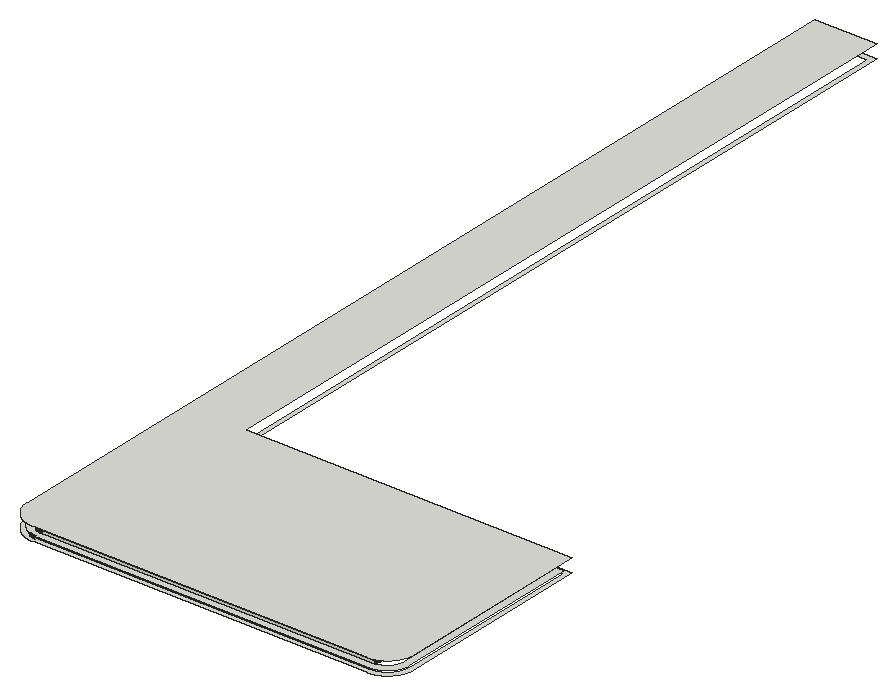
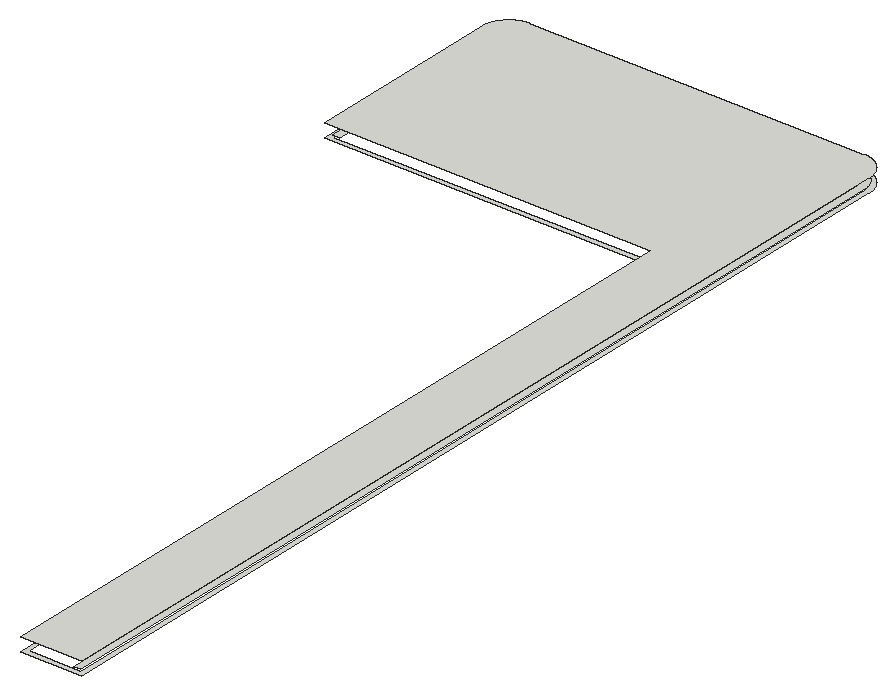
# SketchUp Ruby script. Lengths in inches.
U = 1.inch
M = Sketchup.active_model
def pt(a) = Geom::Point3d.new(a.map { |v| v * U })
def face(e, loops, mat)
  f = e.add_face(loops[0].map { |a| pt(a) })
  loops[1..].each { |l| e.add_face(l.map { |a| pt(a) }).erase! }
  f.material = f.back_material = mat if mat
  f
end
# faces: each face lists its corners as indices into pts; further lists are holes
def faces(e, pts, list, mat = nil) = list.each { |f| face(e, (f[0].is_a?(Array) ? f : [f]).map { |l| l.map { |i| pts[i] } }, mat) }
# xy, xz, yz: faces in a plane at the given z, y or x. An outline is a flat list of corners, or four numbers for a rectangle; further outlines are holes
def ring(l) = l.size == 4 ? [[l[0], l[1]], [l[2], l[1]], [l[2], l[3]], [l[0], l[3]]] : l.each_slice(2).to_a
def flat(e, list, mat, &to3) = list.each { |f| face(e, (f[0].is_a?(Array) ? f : [f]).map { |l| ring(l).map { |u, v| to3.(u, v) } }, mat) }
def xy(e, z, list, mat = nil) = flat(e, list, mat) { |x, y| [x, y, z] }
def xz(e, y, list, mat = nil) = flat(e, list, mat) { |x, z| [x, y, z] }
def yz(e, x, list, mat = nil) = flat(e, list, mat) { |y, z| [x, y, z] }
def lines(e, pts, list) = list.each { |a, b| e.add_line(pt(pts[a]), pt(pts[b])) }
# prism: a flat outline (further loops are holes) pulled along v
def prism(e, loops, v, mat = nil)
  f = face(e, loops, mat); d = Geom::Vector3d.new(v.map { |x| x * U })
  f.pushpull(f.normal.samedirection?(d) ? d.length : -d.length)
end
def box(e, o, s, mat = nil) = prism(e, [[o, [o[0] + s[0], o[1], o[2]], [o[0] + s[0], o[1] + s[1], o[2]], [o[0], o[1] + s[1], o[2]]]], [0, 0, s[2]], mat)
def at(x, y, z, deg = 0) = Geom::Transformation.translation(pt([x, y, z])) * Geom::Transformation.rotation(ORIGIN, Z_AXIS, deg.degrees)
def axes(o, x, y, z) = Geom::Transformation.new([*x, 0, *y, 0, *z, 0, *pt(o).to_a, 1])
def part(name) = M.definitions.add(name)
# library, detail: a bought-in or finely detailed component or shape, given as its bounding box
def library(name, o, s) = part(name).tap { |d| box(d.entities, o, s) }
def detail(e, o, s) = box(e.add_group.entities, o, s)
def put(e, d, t, mat = nil) = e.add_instance(d, t).tap { |i| i.material = mat if mat }
def group(e, t, mat = nil) = e.add_group.tap { |g| g.transformation = t; g.material = mat if mat }.entities
root = M.entities
xy(root,246,[[[29.6875,227,29.53,227.01,29.37,227.02,29.22,227.03,28.9,227.05,28.75,227.07,28.59,227.08,28.43,227.1,28.28,227.125,28.12,227.15,27.97,227.17,27.8125,227.2,27.66,227.23,27.51,227.26,27.35,227.3,27.2,227.33,27.05,227.37,26.89,227.41,26.59,227.49,26.14,227.64,25.99,227.6875,25.85,227.74,25.7,227.8,25.55,227.85,25.41,227.91,25.26,227.97,25.12,228.04,24.98,228.1,24.83,228.17,24.27,228.45,24.14,228.53,24,228.61,23.86,228.6875,23.73,228.77,23.6,228.85,23.46,228.9375,23.33,229.02,23.07,229.2,22.95,229.29,22.82,229.38,22.69,229.48,22.57,229.58,22.45,229.67,22.33,229.77,22.09,229.98,21.97,230.08,21.85,230.1875,21.74,230.3,21.625,230.4,21.51,230.51,21.4,230.625,21.3,230.74,21.1875,230.85,21.08,230.97,20.98,231.09,20.77,231.33,20.67,231.45,20.58,231.57,20.48,231.69,20.38,231.82,20.29,231.95,20.2,232.07,20.02,232.33,19.9375,232.46,19.85,232.6,19.77,232.73,19.6875,232.86,19.61,233,19.53,233.14,19.45,233.27,19.17,233.83,19.1,233.98,19.04,234.12,18.97,234.26,18.91,234.41,18.85,234.55,18.8,234.7,18.74,234.85,18.6875,234.99,18.64,235.14,18.49,235.59,18.41,235.89,18.37,236.05,18.33,236.2,18.3,236.35,18.26,236.51,18.23,236.66,18.2,236.8125,18.17,236.97,18.15,237.12,18.125,237.28,18.1,237.43,18.08,237.59,18.07,237.75,18.05,237.9,18.03,238.22,18.02,238.37,18.01,238.53,18,238.6875,18,674,45,674,45,325.75,189,325.75,189,238.6875,188.99,238.53,188.98,238.37,188.97,238.22,188.95,237.9,188.93,237.75,188.92,237.59,188.9,237.43,188.875,237.28,188.85,237.12,188.83,236.97,188.8,236.8125,188.77,236.66,188.74,236.51,188.7,236.35,188.67,236.2,188.63,236.05,188.59,235.89,188.51,235.59,188.36,235.14,188.3125,234.99,188.26,234.85,188.2,234.7,188.15,234.55,188.09,234.41,188.03,234.26,187.96,234.12,187.9,233.98,187.83,233.83,187.55,233.27,187.47,233.14,187.39,233,187.3125,232.86,187.23,232.73,187.15,232.6,187.0625,232.46,186.98,232.33,186.8,232.07,186.71,231.95,186.62,231.82,186.52,231.69,186.42,231.57,186.33,231.45,186.23,231.33,186.02,231.09,185.92,230.97,185.8125,230.85,185.7,230.74,185.6,230.625,185.49,230.51,185.375,230.4,185.26,230.3,185.15,230.1875,185.03,230.08,184.91,229.98,184.67,229.77,184.55,229.67,184.43,229.58,184.31,229.48,184.18,229.38,184.05,229.29,183.93,229.2,183.67,229.02,183.54,228.9375,183.4,228.85,183.27,228.77,183.14,228.6875,183,228.61,182.86,228.53,182.73,228.45,182.17,228.17,182.02,228.1,181.88,228.04,181.74,227.97,181.59,227.91,181.45,227.85,181.3,227.8,181.15,227.74,181.01,227.6875,180.86,227.64,180.41,227.49,180.11,227.41,179.95,227.37,179.8,227.33,179.65,227.3,179.49,227.26,179.34,227.23,179.1875,227.2,179.03,227.17,178.88,227.15,178.72,227.125,178.57,227.1,178.41,227.08,178.25,227.07,178.1,227.05,177.78,227.03,177.63,227.02,177.47,227.01,177.3125,227],[29.74,229,177.26,229,177.39,229.01,177.52,229.01,177.78,229.03,177.92,229.04,178.05,229.05,178.31,229.09,178.43,229.1,178.5625,229.125,178.69,229.14,178.82,229.17,178.95,229.19,179.21,229.25,179.33,229.28,179.59,229.34,179.71,229.375,179.84,229.41,179.97,229.45,180.21,229.53,180.34,229.57,180.46,229.62,180.58,229.66,180.71,229.71,180.83,229.76,180.95,229.8125,181.07,229.86,181.1875,229.92,181.31,229.97,181.42,230.03,181.66,230.15,181.77,230.21,181.89,230.28,182,230.34,182.11,230.41,182.22,230.47,182.34,230.54,182.45,230.61,182.56,230.69,182.66,230.76,182.77,230.83,182.88,230.91,182.98,230.99,183.09,231.07,183.29,231.23,183.39,231.3125,183.49,231.4,183.59,231.48,183.79,231.66,183.88,231.75,183.98,231.84,184.16,232.02,184.25,232.12,184.34,232.21,184.52,232.41,184.6,232.51,184.6875,232.61,184.77,232.71,184.93,232.91,185.01,233.02,185.09,233.12,185.17,233.23,185.24,233.34,185.31,233.44,185.39,233.55,185.46,233.66,185.53,233.78,185.59,233.89,185.66,234,185.72,234.11,185.79,234.23,185.85,234.34,185.97,234.58,186.03,234.69,186.08,234.8125,186.14,234.93,186.1875,235.05,186.24,235.17,186.29,235.29,186.34,235.42,186.38,235.54,186.43,235.66,186.47,235.79,186.55,236.03,186.59,236.16,186.625,236.29,186.66,236.41,186.72,236.67,186.75,236.79,186.81,237.05,186.83,237.18,186.86,237.31,186.875,237.4375,186.9,237.57,186.91,237.69,186.95,237.95,186.96,238.08,186.97,238.22,186.99,238.48,186.99,238.61,187,238.74,187,323.75,43,323.75,43,672,20,672,20,238.74,20.01,238.61,20.01,238.48,20.03,238.22,20.04,238.08,20.05,237.95,20.09,237.69,20.1,237.57,20.125,237.4375,20.14,237.31,20.17,237.18,20.19,237.05,20.25,236.79,20.28,236.67,20.34,236.41,20.375,236.29,20.41,236.16,20.45,236.03,20.53,235.79,20.57,235.66,20.62,235.54,20.66,235.42,20.71,235.29,20.76,235.17,20.8125,235.05,20.86,234.93,20.92,234.8125,20.97,234.69,21.03,234.58,21.15,234.34,21.21,234.23,21.28,234.11,21.34,234,21.41,233.89,21.47,233.78,21.54,233.66,21.61,233.55,21.69,233.44,21.76,233.34,21.83,233.23,21.91,233.12,21.99,233.02,22.07,232.91,22.23,232.71,22.3125,232.61,22.4,232.51,22.48,232.41,22.66,232.21,22.75,232.12,22.84,232.02,23.02,231.84,23.12,231.75,23.21,231.66,23.41,231.48,23.51,231.4,23.61,231.3125,23.71,231.23,23.91,231.07,24.02,230.99,24.12,230.91,24.23,230.83,24.34,230.76,24.44,230.69,24.55,230.61,24.66,230.54,24.78,230.47,24.89,230.41,25,230.34,25.11,230.28,25.23,230.21,25.34,230.15,25.58,230.03,25.69,229.97,25.8125,229.92,25.93,229.86,26.05,229.8125,26.17,229.76,26.29,229.71,26.42,229.66,26.54,229.62,26.66,229.57,26.79,229.53,27.03,229.45,27.16,229.41,27.29,229.375,27.41,229.34,27.67,229.28,27.79,229.25,28.05,229.19,28.18,229.17,28.31,229.14,28.4375,229.125,28.57,229.1,28.69,229.09,28.95,229.05,29.08,229.04,29.22,229.03,29.48,229.01,29.61,229.01]]])
xy(root,247,[[29.74,229,29.61,229.01,29.48,229.01,29.22,229.03,29.08,229.04,28.95,229.05,28.69,229.09,28.57,229.1,28.4375,229.125,28.31,229.14,28.18,229.17,28.05,229.19,27.79,229.25,27.67,229.28,27.41,229.34,27.29,229.375,27.16,229.41,27.03,229.45,26.79,229.53,26.66,229.57,26.54,229.62,26.42,229.66,26.29,229.71,26.17,229.76,26.05,229.8125,25.93,229.86,25.8125,229.92,25.69,229.97,25.58,230.03,25.34,230.15,25.23,230.21,25.11,230.28,25,230.34,24.89,230.41,24.78,230.47,24.66,230.54,24.55,230.61,24.44,230.69,24.34,230.76,24.23,230.83,24.12,230.91,24.02,230.99,23.91,231.07,23.71,231.23,23.61,231.3125,23.51,231.4,23.41,231.48,23.21,231.66,23.12,231.75,23.02,231.84,22.84,232.02,22.75,232.12,22.66,232.21,22.48,232.41,22.4,232.51,22.3125,232.61,22.23,232.71,22.07,232.91,21.99,233.02,21.91,233.12,21.83,233.23,21.76,233.34,21.69,233.44,21.61,233.55,21.54,233.66,21.47,233.78,21.41,233.89,21.34,234,21.28,234.11,21.21,234.23,21.15,234.34,21.03,234.58,20.97,234.69,20.92,234.8125,20.86,234.93,20.8125,235.05,20.76,235.17,20.71,235.29,20.66,235.42,20.62,235.54,20.57,235.66,20.53,235.79,20.45,236.03,20.41,236.16,20.375,236.29,20.34,236.41,20.28,236.67,20.25,236.79,20.19,237.05,20.17,237.18,20.14,237.31,20.125,237.4375,20.1,237.57,20.09,237.69,20.05,237.95,20.04,238.08,20.03,238.22,20.01,238.48,20.01,238.61,20,238.74,20,672,23,672,23,238.82,23.01,238.73,23.01,238.54,23.07,238,23.09,237.9,23.1,237.81,23.12,237.72,23.13,237.63,23.15,237.54,23.17,237.46,23.19,237.37,23.22,237.28,23.24,237.1875,23.26,237.1,23.29,237.01,23.31,236.92,23.34,236.84,23.4,236.66,23.43,236.58,23.46,236.49,23.5,236.41,23.53,236.32,23.57,236.24,23.61,236.15,23.64,236.07,23.68,235.99,23.72,235.9,23.76,235.82,23.81,235.74,23.89,235.58,23.9375,235.5,23.98,235.42,24.08,235.26,24.13,235.1875,24.18,235.11,24.23,235.04,24.28,234.96,24.34,234.89,24.39,234.8125,24.45,234.74,24.5,234.67,24.56,234.59,24.74,234.38,24.8,234.32,24.92,234.18,24.99,234.12,25.05,234.05,25.12,233.99,25.18,233.92,25.32,233.8,25.38,233.74,25.59,233.56,25.67,233.5,25.74,233.45,25.8125,233.39,25.89,233.34,25.96,233.28,26.04,233.23,26.11,233.18,26.1875,233.13,26.26,233.08,26.42,232.98,26.5,232.9375,26.58,232.89,26.74,232.81,26.82,232.76,26.9,232.72,26.99,232.68,27.07,232.64,27.15,232.61,27.24,232.57,27.32,232.53,27.41,232.5,27.49,232.46,27.58,232.43,27.66,232.4,27.84,232.34,27.92,232.31,28.01,232.29,28.1,232.26,28.1875,232.24,28.28,232.22,28.37,232.19,28.46,232.17,28.54,232.15,28.63,232.13,28.72,232.12,28.81,232.1,28.9,232.09,29,232.07,29.54,232.01,29.73,232.01,29.82,232,177.18,232,177.27,232.01,177.46,232.01,178,232.07,178.1,232.09,178.19,232.1,178.28,232.12,178.37,232.13,178.46,232.15,178.54,232.17,178.63,232.19,178.72,232.22,178.8125,232.24,178.9,232.26,178.99,232.29,179.08,232.31,179.16,232.34,179.34,232.4,179.42,232.43,179.51,232.46,179.59,232.5,179.68,232.53,179.76,232.57,179.85,232.61,179.93,232.64,180.01,232.68,180.1,232.72,180.18,232.76,180.26,232.81,180.42,232.89,180.5,232.9375,180.58,232.98,180.74,233.08,180.8125,233.13,180.89,233.18,180.96,233.23,181.04,233.28,181.11,233.34,181.1875,233.39,181.26,233.45,181.33,233.5,181.41,233.56,181.62,233.74,181.68,233.8,181.82,233.92,181.88,233.99,181.95,234.05,182.01,234.12,182.08,234.18,182.2,234.32,182.26,234.38,182.44,234.59,182.5,234.67,182.55,234.74,182.61,234.8125,182.66,234.89,182.72,234.96,182.77,235.04,182.82,235.11,182.87,235.1875,182.92,235.26,183.02,235.42,183.0625,235.5,183.11,235.58,183.19,235.74,183.24,235.82,183.28,235.9,183.32,235.99,183.36,236.07,183.39,236.15,183.43,236.24,183.47,236.32,183.5,236.41,183.54,236.49,183.57,236.58,183.6,236.66,183.66,236.84,183.69,236.92,183.71,237.01,183.74,237.1,183.76,237.1875,183.78,237.28,183.81,237.37,183.83,237.46,183.85,237.54,183.87,237.63,183.88,237.72,183.9,237.81,183.91,237.9,183.93,238,183.99,238.54,183.99,238.73,184,238.82,184,323.75,187,323.75,187,238.74,186.99,238.61,186.99,238.48,186.97,238.22,186.96,238.08,186.95,237.95,186.91,237.69,186.9,237.57,186.875,237.4375,186.86,237.31,186.83,237.18,186.81,237.05,186.75,236.79,186.72,236.67,186.66,236.41,186.625,236.29,186.59,236.16,186.55,236.03,186.47,235.79,186.43,235.66,186.38,235.54,186.34,235.42,186.29,235.29,186.24,235.17,186.1875,235.05,186.14,234.93,186.08,234.8125,186.03,234.69,185.97,234.58,185.85,234.34,185.79,234.23,185.72,234.11,185.66,234,185.59,233.89,185.53,233.78,185.46,233.66,185.39,233.55,185.31,233.44,185.24,233.34,185.17,233.23,185.09,233.12,185.01,233.02,184.93,232.91,184.77,232.71,184.6875,232.61,184.6,232.51,184.52,232.41,184.34,232.21,184.25,232.12,184.16,232.02,183.98,231.84,183.88,231.75,183.79,231.66,183.59,231.48,183.49,231.4,183.39,231.3125,183.29,231.23,183.09,231.07,182.98,230.99,182.88,230.91,182.77,230.83,182.66,230.76,182.56,230.69,182.45,230.61,182.34,230.54,182.22,230.47,182.11,230.41,182,230.34,181.89,230.28,181.77,230.21,181.66,230.15,181.42,230.03,181.31,229.97,181.1875,229.92,181.07,229.86,180.95,229.8125,180.83,229.76,180.71,229.71,180.58,229.66,180.46,229.62,180.34,229.57,180.21,229.53,179.97,229.45,179.84,229.41,179.71,229.375,179.59,229.34,179.33,229.28,179.21,229.25,178.95,229.19,178.82,229.17,178.69,229.14,178.5625,229.125,178.43,229.1,178.31,229.09,178.05,229.05,177.92,229.04,177.78,229.03,177.52,229.01,177.39,229.01,177.26,229]])
xy(root,252,[[29.6875,227,177.3125,227,177.47,227.01,177.63,227.02,177.78,227.03,178.1,227.05,178.25,227.07,178.41,227.08,178.57,227.1,178.72,227.125,178.88,227.15,179.03,227.17,179.1875,227.2,179.34,227.23,179.49,227.26,179.65,227.3,179.8,227.33,179.95,227.37,180.11,227.41,180.41,227.49,180.86,227.64,181.01,227.6875,181.15,227.74,181.3,227.8,181.45,227.85,181.59,227.91,181.74,227.97,181.88,228.04,182.02,228.1,182.17,228.17,182.73,228.45,182.86,228.53,183,228.61,183.14,228.6875,183.27,228.77,183.4,228.85,183.54,228.9375,183.67,229.02,183.93,229.2,184.05,229.29,184.18,229.38,184.31,229.48,184.43,229.58,184.55,229.67,184.67,229.77,184.91,229.98,185.03,230.08,185.15,230.1875,185.26,230.3,185.375,230.4,185.49,230.51,185.6,230.625,185.7,230.74,185.8125,230.85,185.92,230.97,186.02,231.09,186.23,231.33,186.33,231.45,186.42,231.57,186.52,231.69,186.62,231.82,186.71,231.95,186.8,232.07,186.98,232.33,187.0625,232.46,187.15,232.6,187.23,232.73,187.3125,232.86,187.39,233,187.47,233.14,187.55,233.27,187.83,233.83,187.9,233.98,187.96,234.12,188.03,234.26,188.09,234.41,188.15,234.55,188.2,234.7,188.26,234.85,188.3125,234.99,188.36,235.14,188.51,235.59,188.59,235.89,188.63,236.05,188.67,236.2,188.7,236.35,188.74,236.51,188.77,236.66,188.8,236.8125,188.83,236.97,188.85,237.12,188.875,237.28,188.9,237.43,188.92,237.59,188.93,237.75,188.95,237.9,188.97,238.22,188.98,238.37,188.99,238.53,189,238.6875,189,325.75,45,325.75,45,674,18,674,18,238.6875,18.01,238.53,18.02,238.37,18.03,238.22,18.05,237.9,18.07,237.75,18.08,237.59,18.1,237.43,18.125,237.28,18.15,237.12,18.17,236.97,18.2,236.8125,18.23,236.66,18.26,236.51,18.3,236.35,18.33,236.2,18.37,236.05,18.41,235.89,18.49,235.59,18.64,235.14,18.6875,234.99,18.74,234.85,18.8,234.7,18.85,234.55,18.91,234.41,18.97,234.26,19.04,234.12,19.1,233.98,19.17,233.83,19.45,233.27,19.53,233.14,19.61,233,19.6875,232.86,19.77,232.73,19.85,232.6,19.9375,232.46,20.02,232.33,20.2,232.07,20.29,231.95,20.38,231.82,20.48,231.69,20.58,231.57,20.67,231.45,20.77,231.33,20.98,231.09,21.08,230.97,21.1875,230.85,21.3,230.74,21.4,230.625,21.51,230.51,21.625,230.4,21.74,230.3,21.85,230.1875,21.97,230.08,22.09,229.98,22.33,229.77,22.45,229.67,22.57,229.58,22.69,229.48,22.82,229.38,22.95,229.29,23.07,229.2,23.33,229.02,23.46,228.9375,23.6,228.85,23.73,228.77,23.86,228.6875,24,228.61,24.14,228.53,24.27,228.45,24.83,228.17,24.98,228.1,25.12,228.04,25.26,227.97,25.41,227.91,25.55,227.85,25.7,227.8,25.85,227.74,25.99,227.6875,26.14,227.64,26.59,227.49,26.89,227.41,27.05,227.37,27.2,227.33,27.35,227.3,27.51,227.26,27.66,227.23,27.8125,227.2,27.97,227.17,28.12,227.15,28.28,227.125,28.43,227.1,28.59,227.08,28.75,227.07,28.9,227.05,29.22,227.03,29.37,227.02,29.53,227.01],[29.6875,227,29.53,227.01,29.37,227.02,29.22,227.03,28.9,227.05,28.75,227.07,28.59,227.08,28.43,227.1,28.28,227.125,28.12,227.15,27.97,227.17,27.8125,227.2,27.66,227.23,27.51,227.26,27.35,227.3,27.2,227.33,27.05,227.37,26.89,227.41,26.59,227.49,26.14,227.64,25.99,227.6875,25.85,227.74,25.7,227.8,25.55,227.85,25.41,227.91,25.26,227.97,25.12,228.04,24.98,228.1,24.83,228.17,24.27,228.45,24.14,228.53,24,228.61,23.86,228.6875,23.73,228.77,23.6,228.85,23.46,228.9375,23.33,229.02,23.07,229.2,22.95,229.29,22.82,229.38,22.69,229.48,22.57,229.58,22.45,229.67,22.33,229.77,22.09,229.98,21.97,230.08,21.85,230.1875,21.74,230.3,21.625,230.4,21.51,230.51,21.4,230.625,21.3,230.74,21.1875,230.85,21.08,230.97,20.98,231.09,20.77,231.33,20.67,231.45,20.58,231.57,20.48,231.69,20.38,231.82,20.29,231.95,20.2,232.07,20.02,232.33,19.9375,232.46,19.85,232.6,19.77,232.73,19.6875,232.86,19.61,233,19.53,233.14,19.45,233.27,19.17,233.83,19.1,233.98,19.04,234.12,18.97,234.26,18.91,234.41,18.85,234.55,18.8,234.7,18.74,234.85,18.6875,234.99,18.64,235.14,18.49,235.59,18.41,235.89,18.37,236.05,18.33,236.2,18.3,236.35,18.26,236.51,18.23,236.66,18.2,236.8125,18.17,236.97,18.15,237.12,18.125,237.28,18.1,237.43,18.08,237.59,18.07,237.75,18.05,237.9,18.03,238.22,18.02,238.37,18.01,238.53,18,238.6875,18,674,45,674,45,325.75,189,325.75,189,238.6875,188.99,238.53,188.98,238.37,188.97,238.22,188.95,237.9,188.93,237.75,188.92,237.59,188.9,237.43,188.875,237.28,188.85,237.12,188.83,236.97,188.8,236.8125,188.77,236.66,188.74,236.51,188.7,236.35,188.67,236.2,188.63,236.05,188.59,235.89,188.51,235.59,188.36,235.14,188.3125,234.99,188.26,234.85,188.2,234.7,188.15,234.55,188.09,234.41,188.03,234.26,187.96,234.12,187.9,233.98,187.83,233.83,187.55,233.27,187.47,233.14,187.39,233,187.3125,232.86,187.23,232.73,187.15,232.6,187.0625,232.46,186.98,232.33,186.8,232.07,186.71,231.95,186.62,231.82,186.52,231.69,186.42,231.57,186.33,231.45,186.23,231.33,186.02,231.09,185.92,230.97,185.8125,230.85,185.7,230.74,185.6,230.625,185.49,230.51,185.375,230.4,185.26,230.3,185.15,230.1875,185.03,230.08,184.91,229.98,184.67,229.77,184.55,229.67,184.43,229.58,184.31,229.48,184.18,229.38,184.05,229.29,183.93,229.2,183.67,229.02,183.54,228.9375,183.4,228.85,183.27,228.77,183.14,228.6875,183,228.61,182.86,228.53,182.73,228.45,182.17,228.17,182.02,228.1,181.88,228.04,181.74,227.97,181.59,227.91,181.45,227.85,181.3,227.8,181.15,227.74,181.01,227.6875,180.86,227.64,180.41,227.49,180.11,227.41,179.95,227.37,179.8,227.33,179.65,227.3,179.49,227.26,179.34,227.23,179.1875,227.2,179.03,227.17,178.88,227.15,178.72,227.125,178.57,227.1,178.41,227.08,178.25,227.07,178.1,227.05,177.78,227.03,177.63,227.02,177.47,227.01,177.3125,227]])
xz(root,232,[[29.82,247,29.91,248],[29.91,247,30,248],[30,247,177,248],[177,247,177.09,248],[177.09,247,177.18,248]])
xz(root,232.01,[[29.54,247,29.63,248],[29.63,247,29.73,248],[177.27,247,177.37,248],[177.37,247,177.46,248]])
xz(root,234,[[29.8,247,29.87,248],[29.87,247,29.93,248],[29.93,247,30,248],[30,247,177,248],[177,247,177.07,248],
  [177.07,247,177.13,248],[177.13,247,177.2,248]])
xz(root,234.01,[[29.67,247,29.74,248],[177.26,247,177.33,248]])
xz(root,234.02,[[29.54,247,29.61,248],[177.39,247,177.46,248]])
xz(root,234.03,[[29.41,247,29.48,248],[177.52,247,177.59,248]])
p = [[29.08,229.04,246],[28.95,229.05,246],[28.95,229.05,247],[29.08,229.04,247],[29.22,229.03,246],[29.22,229.03,247],
  [29.35,229.02,246],[29.35,229.02,247],[28.31,229.14,246],[28.18,229.17,246],[28.18,229.17,247],[28.31,229.14,247],
  [28.4375,229.125,246],[28.4375,229.125,247],[28.57,229.1,246],[28.57,229.1,247],[28.69,229.09,246],[28.69,229.09,247],
  [28.82,229.07,246],[28.82,229.07,247],[27.79,229.25,246],[27.67,229.28,246],[27.67,229.28,247],[27.79,229.25,247],
  [27.92,229.22,246],[27.92,229.22,247],[28.05,229.19,246],[28.05,229.19,247],[27.41,229.34,246],[27.29,229.375,246],
  [27.29,229.375,247],[27.41,229.34,247],[27.54,229.31,246],[27.54,229.31,247],[27.03,229.45,246],[26.91,229.49,246],
  [26.91,229.49,247],[27.03,229.45,247],[27.16,229.41,246],[27.16,229.41,247],[26.79,229.53,246],[26.66,229.57,246],
  [26.66,229.57,247],[26.79,229.53,247],[26.54,229.62,246],[26.54,229.62,247],[29.18,232.05,248],[29.18,232.05,247],
  [29.09,232.06,247],[29.09,232.06,248],[29.27,232.04,248],[29.27,232.04,247],[29.36,232.03,248],[29.36,232.03,247],
  [29.45,232.02,248],[29.45,232.02,247],[29.54,232.01,248],[29.54,232.01,247],[29.82,232,248],[29.82,232,247],
  [29.73,232.01,247],[29.73,232.01,248],[177.27,232.01,248],[177.27,232.01,247],[177.18,232,247],[177.18,232,248],
  [177.55,232.02,248],[177.55,232.02,247],[177.46,232.01,247],[177.46,232.01,248],[177.64,232.03,248],[177.64,232.03,247],
  [177.73,232.04,248],[177.73,232.04,247],[28.63,232.13,248],[28.63,232.13,247],[28.54,232.15,247],[28.54,232.15,248],
  [28.72,232.12,248],[28.72,232.12,247],[28.81,232.1,248],[28.81,232.1,247],[28.9,232.09,248],[28.9,232.09,247],
  [29,232.07,248],[29,232.07,247],[28.1875,232.24,248],[28.1875,232.24,247],[28.1,232.26,247],[28.1,232.26,248],
  [28.28,232.22,248],[28.28,232.22,247],[28.37,232.19,248],[28.37,232.19,247],[28.46,232.17,248],[28.46,232.17,247],
  [27.84,232.34,248],[27.84,232.34,247],[27.75,232.37,247],[27.75,232.37,248],[27.92,232.31,248],[27.92,232.31,247],
  [28.01,232.29,248],[28.01,232.29,247],[27.58,232.43,248],[27.58,232.43,247],[27.49,232.46,247],[27.49,232.46,248],
  [27.66,232.4,248],[27.66,232.4,247],[27.32,232.53,248],[27.32,232.53,247],[27.24,232.57,247],[27.24,232.57,248],
  [27.41,232.5,248],[27.41,232.5,247],[27.07,232.64,248],[27.07,232.64,247],[26.99,232.68,247],[26.99,232.68,248],
  [27.15,232.61,248],[27.15,232.61,247],[26.9,232.72,248],[26.9,232.72,247],[26.82,232.76,247],[26.82,232.76,248],
  [26.66,232.85,248],[26.66,232.85,247],[26.58,232.89,247],[26.58,232.89,248],[26.74,232.81,248],[26.74,232.81,247],
  [29.28,234.05,247],[29.35,234.04,247],[29.35,234.04,248],[29.28,234.05,248],[29.41,234.03,247],[29.41,234.03,248],
  [29.48,234.03,247],[29.54,234.02,247],[29.54,234.02,248],[29.48,234.03,248],[29.61,234.02,247],[29.67,234.01,247],
  [29.67,234.01,248],[29.61,234.02,248],[29.74,234.01,247],[29.8,234,247],[29.8,234,248],[29.74,234.01,248],
  [177.2,234,247],[177.26,234.01,247],[177.26,234.01,248],[177.2,234,248],[177.33,234.01,247],[177.39,234.02,247],
  [177.39,234.02,248],[177.33,234.01,248],[177.46,234.02,247],[177.52,234.03,247],[177.52,234.03,248],[177.46,234.02,248],
  [177.59,234.03,247],[177.65,234.04,247],[177.65,234.04,248],[177.59,234.03,248],[177.72,234.05,247],[177.72,234.05,248],
  [28.77,234.15,247],[28.83,234.14,247],[28.83,234.14,248],[28.77,234.15,248],[28.9,234.125,247],[28.9,234.125,248],
  [28.96,234.11,247],[28.96,234.11,248],[29.02,234.1,247],[29.02,234.1,248],[29.09,234.08,247],[29.09,234.08,248],
  [29.15,234.07,247],[29.15,234.07,248],[29.22,234.0625,247],[29.22,234.0625,248],[177.78,234.0625,247],[177.78,234.0625,248],
  [28.39,234.27,247],[28.45,234.24,247],[28.45,234.24,248],[28.39,234.27,248],[28.52,234.22,247],[28.52,234.22,248],
  [28.58,234.21,247],[28.58,234.21,248],[28.64,234.1875,247],[28.64,234.1875,248],[28.71,234.17,247],[28.71,234.17,248],
  [28.15,234.36,247],[28.21,234.33,247],[28.21,234.33,248],[28.15,234.36,248],[28.27,234.31,247],[28.27,234.31,248],
  [28.33,234.29,247],[28.33,234.29,248],[27.91,234.46,247],[27.97,234.43,247],[27.97,234.43,248],[27.91,234.46,248],
  [28.03,234.41,247],[28.03,234.41,248],[28.09,234.38,247],[28.09,234.38,248],[27.67,234.58,247],[27.73,234.54,247],
  [27.73,234.54,248],[27.67,234.58,248],[27.79,234.52,247],[27.79,234.52,248],[27.85,234.49,247],[27.85,234.49,248],
  [27.5,234.67,247],[27.56,234.64,247],[27.56,234.64,248],[27.5,234.67,248],[27.61,234.61,247],[27.61,234.61,248],
  [27.33,234.77,247],[27.39,234.74,247],[27.39,234.74,248],[27.33,234.77,248],[27.44,234.7,247],[27.44,234.7,248],
  [27.17,234.88,247],[27.22,234.84,247],[27.22,234.84,248],[27.17,234.88,248],[27.28,234.81,247],[27.28,234.81,248],
  [27.0625,234.95,247],[27.11,234.92,247],[27.11,234.92,248],[27.0625,234.95,248],[26.9,235.07,247],[26.96,235.03,247],
  [26.96,235.03,248],[26.9,235.07,248],[27.01,234.99,247],[27.01,234.99,248],[26.8,235.16,247],[26.85,235.11,247],
  [26.85,235.11,248],[26.8,235.16,248],[26.65,235.28,247],[26.7,235.24,247],[26.7,235.24,248],[26.65,235.28,248],
  [26.75,235.2,247],[26.75,235.2,248],[26.61,235.33,247],[26.61,235.33,248],[177.78,229.09,246],[177.65,229.08,246],
  [177.52,229.07,246],[177.39,229.0625,246],[177.26,229.06,246],[177.13,229.06,246],[177,229.05,246]]
faces(root,p,[[0,1,2,3],[4,0,3,5],[6,4,5,7],[8,9,10,11],[12,8,11,13],[14,12,13,15],[16,14,15,17],[18,16,17,19],
  [1,18,19,2],[20,21,22,23],[24,20,23,25],[26,24,25,27],[9,26,27,10],[28,29,30,31],[32,28,31,33],[21,32,33,22],
  [34,35,36,37],[38,34,37,39],[29,38,39,30],[40,41,42,43],[35,40,43,36],[41,44,45,42],[46,47,48,49],[50,51,47,46],
  [52,53,51,50],[54,55,53,52],[56,57,55,54],[58,59,60,61],[62,63,64,65],[66,67,68,69],[70,71,67,66],[72,73,71,70],
  [74,75,76,77],[78,79,75,74],[80,81,79,78],[82,83,81,80],[84,85,83,82],[49,48,85,84],[86,87,88,89],[90,91,87,86],
  [92,93,91,90],[94,95,93,92],[77,76,95,94],[96,97,98,99],[100,101,97,96],[102,103,101,100],[89,88,103,102],[104,105,106,107],
  [108,109,105,104],[99,98,109,108],[110,111,112,113],[114,115,111,110],[107,106,115,114],[116,117,118,119],[120,121,117,116],[113,112,121,120],
  [122,123,124,125],[119,118,123,122],[126,127,128,129],[130,131,127,126],[125,124,131,130],[132,133,134,135],[133,136,137,134],[138,139,140,141],
  [142,143,144,145],[146,147,148,149],[150,151,152,153],[154,155,156,157],[158,159,160,161],[162,163,164,165],[163,166,167,164],[168,169,170,171],
  [169,172,173,170],[172,174,175,173],[174,176,177,175],[176,178,179,177],[178,180,181,179],[180,182,183,181],[182,132,135,183],[166,184,185,167],
  [186,187,188,189],[187,190,191,188],[190,192,193,191],[192,194,195,193],[194,196,197,195],[196,168,171,197],[198,199,200,201],[199,202,203,200],
  [202,204,205,203],[204,186,189,205],[206,207,208,209],[207,210,211,208],[210,212,213,211],[212,198,201,213],[214,215,216,217],[215,218,219,216],
  [218,220,221,219],[220,206,209,221],[222,223,224,225],[223,226,227,224],[226,214,217,227],[228,229,230,231],[229,232,233,230],[232,222,225,233],
  [234,235,236,237],[235,238,239,236],[238,228,231,239],[240,241,242,243],[241,234,237,242],[244,245,246,247],[245,248,249,246],[248,240,243,249],
  [250,251,252,253],[251,244,247,252],[254,255,256,257],[255,258,259,256],[258,250,253,259],[260,254,257,261]])
lines(root,p,[[262,263],[263,264],[264,265],[265,266],[266,267],[267,268]])
